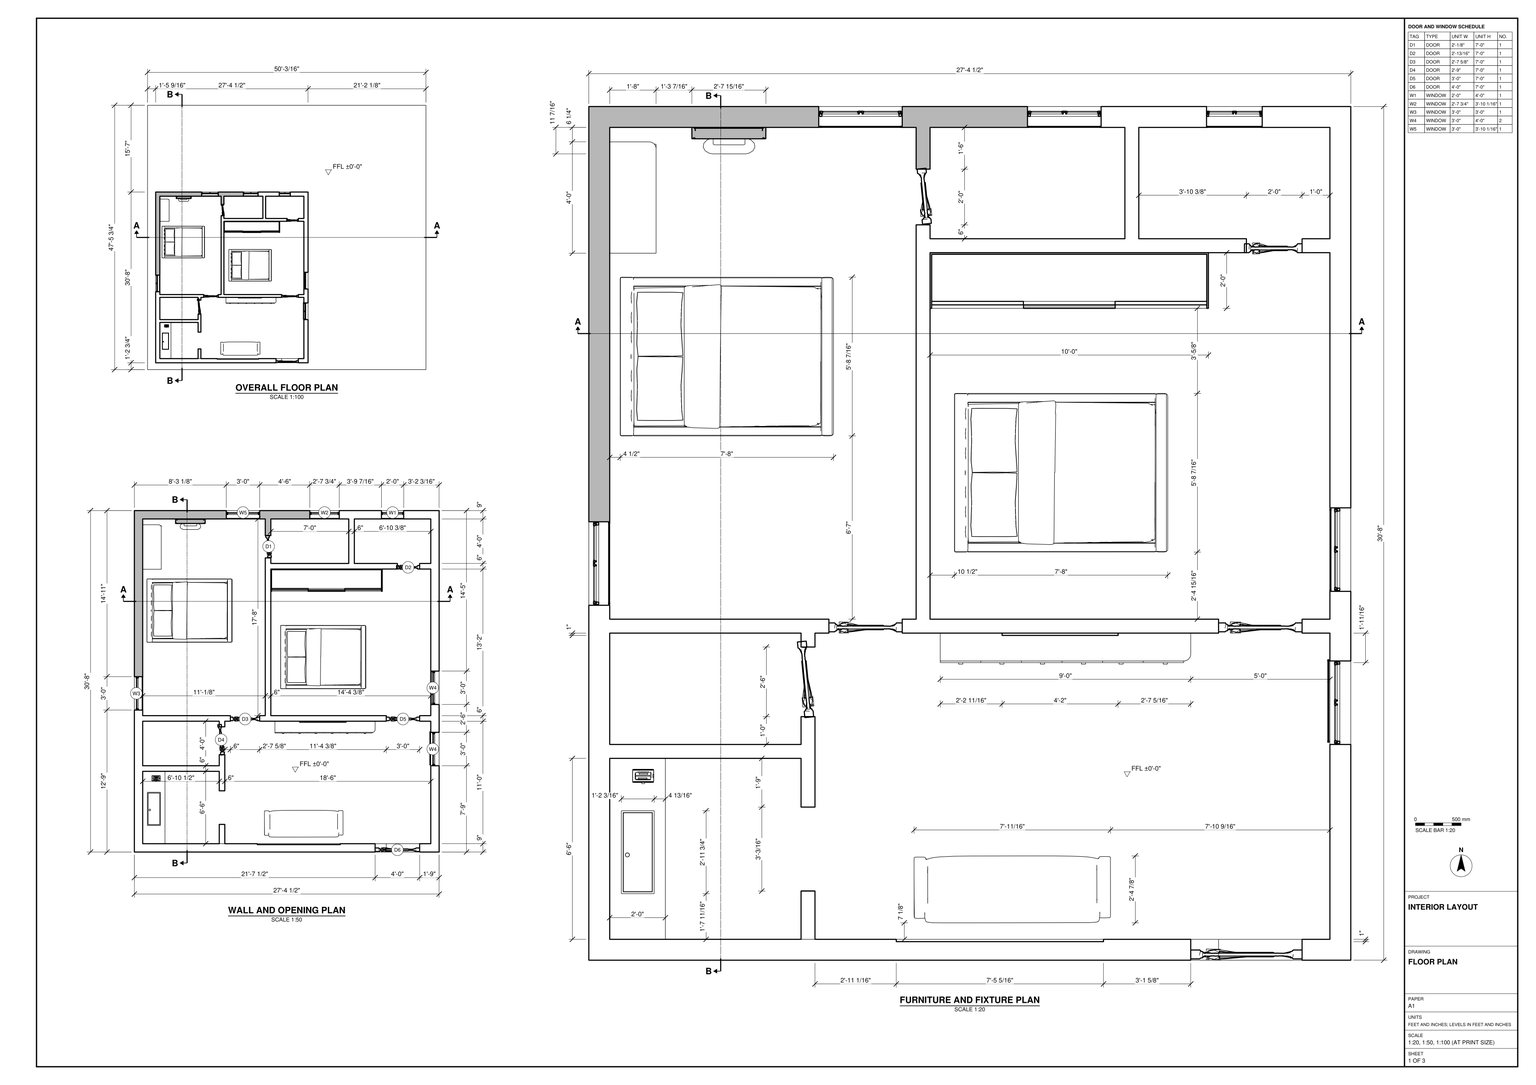
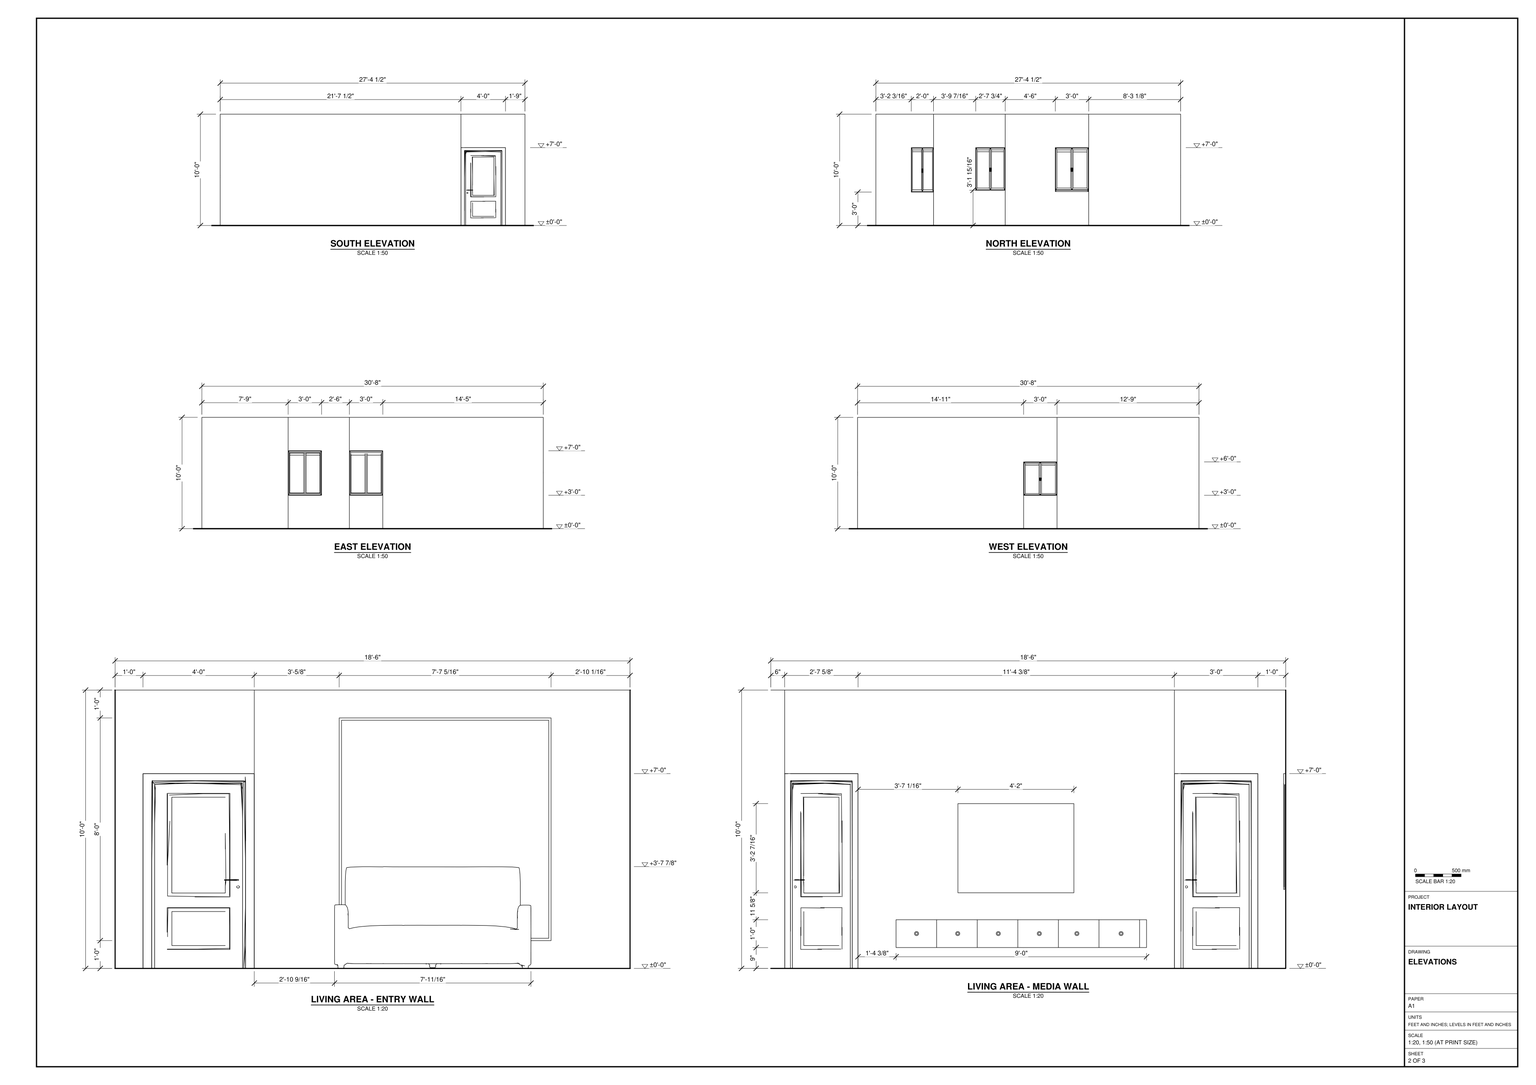
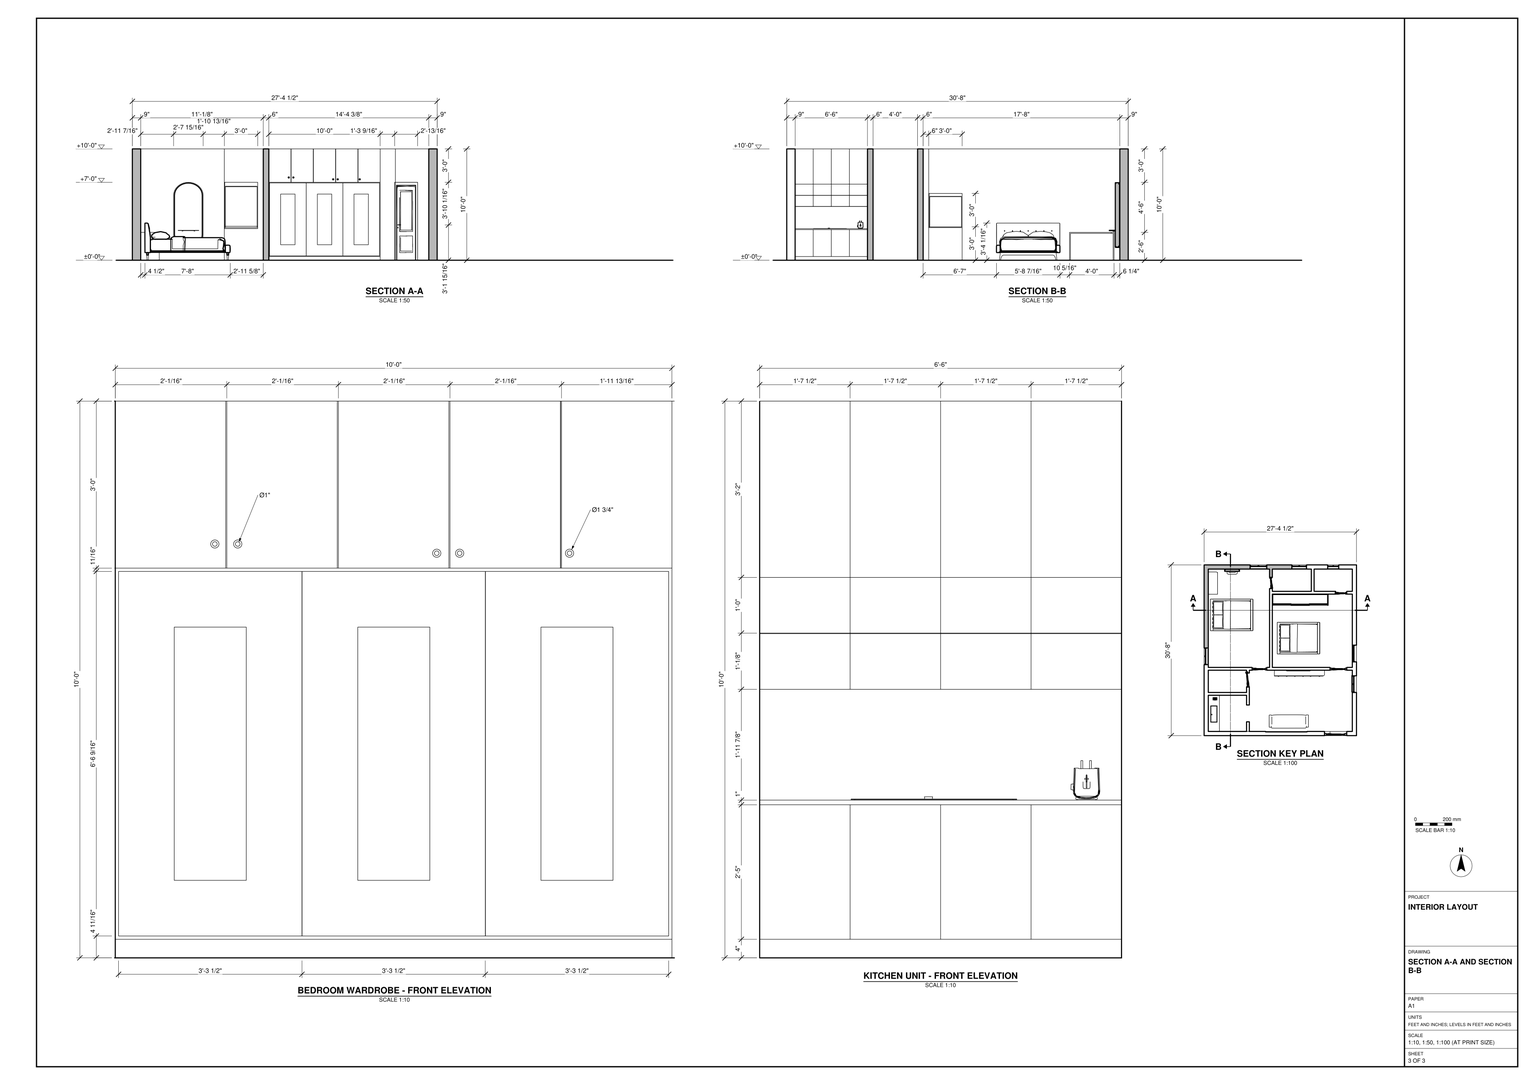
Build the interior in SketchUp from task_files/diagram_01.pdf. Work in feet and inches. The overall model measures 50'-3/16" east to west by 47'-5 3/4" north to south and is 10'-0" high. Set the finished floor at ±0'-0". Use the overall floor plan to position the 27'-4 1/2" by 30'-8" enclosure on the larger floor area; the enclosure and the floor have different footprints.

Build the 9" perimeter walls and 6" internal partitions as drawn. Lay out the two bedrooms, the small enclosed spaces and the living area with its adjoining kitchen. Use the plan and schedule for door and window sizes and positions, and the elevations for sill and head heights.

Place a platform bed in each bedroom with its head to the west. Use the joinery elevations to model the wardrobe in the east bedroom and the kitchen unit along the west wall, including cabinet divisions, the worktop and the cooktop. Place the sofa against the entry wall, with the wall panel behind it, facing the media unit between the bedroom doors. Decor and loose items, including countertop appliances, may be any suitable library components.

Keep shell elements and individual furniture and joinery pieces in separate groups or components, and use components for repeated parts. Save one SketchUp model as output_files/furnished_two_bedroom_interior_with_built_in_joinery.skp.

# SketchUp Ruby script. Lengths in inches.
U = 1.inch
M = Sketchup.active_model
def pt(a) = Geom::Point3d.new(a.map { |v| v * U })
def face(e, loops, mat)
  f = e.add_face(loops[0].map { |a| pt(a) })
  loops[1..].each { |l| e.add_face(l.map { |a| pt(a) }).erase! }
  f.material = f.back_material = mat if mat
  f
end
# faces: each face lists its corners as indices into pts; further lists are holes
def faces(e, pts, list, mat = nil) = list.each { |f| face(e, (f[0].is_a?(Array) ? f : [f]).map { |l| l.map { |i| pts[i] } }, mat) }
# xy, xz, yz: faces in a plane at the given z, y or x. An outline is a flat list of corners, or four numbers for a rectangle; further outlines are holes
def ring(l) = l.size == 4 ? [[l[0], l[1]], [l[2], l[1]], [l[2], l[3]], [l[0], l[3]]] : l.each_slice(2).to_a
def flat(e, list, mat, &to3) = list.each { |f| face(e, (f[0].is_a?(Array) ? f : [f]).map { |l| ring(l).map { |u, v| to3.(u, v) } }, mat) }
def xy(e, z, list, mat = nil) = flat(e, list, mat) { |x, y| [x, y, z] }
def xz(e, y, list, mat = nil) = flat(e, list, mat) { |x, z| [x, y, z] }
def yz(e, x, list, mat = nil) = flat(e, list, mat) { |y, z| [x, y, z] }
def lines(e, pts, list) = list.each { |a, b| e.add_line(pt(pts[a]), pt(pts[b])) }
# prism: a flat outline (further loops are holes) pulled along v
def prism(e, loops, v, mat = nil)
  f = face(e, loops, mat); d = Geom::Vector3d.new(v.map { |x| x * U })
  f.pushpull(f.normal.samedirection?(d) ? d.length : -d.length)
end
def box(e, o, s, mat = nil) = prism(e, [[o, [o[0] + s[0], o[1], o[2]], [o[0] + s[0], o[1] + s[1], o[2]], [o[0], o[1] + s[1], o[2]]]], [0, 0, s[2]], mat)
def at(x, y, z, deg = 0) = Geom::Transformation.translation(pt([x, y, z])) * Geom::Transformation.rotation(ORIGIN, Z_AXIS, deg.degrees)
def axes(o, x, y, z) = Geom::Transformation.new([*x, 0, *y, 0, *z, 0, *pt(o).to_a, 1])
def part(name) = M.definitions.add(name)
# library, detail: a bought-in or finely detailed component or shape, given as its bounding box
def library(name, o, s) = part(name).tap { |d| box(d.entities, o, s) }
def detail(e, o, s) = box(e.add_group.entities, o, s)
def put(e, d, t, mat = nil) = e.add_instance(d, t).tap { |i| i.material = mat if mat }
def group(e, t, mat = nil) = e.add_group.tap { |g| g.transformation = t; g.material = mat if mat }.entities
root = M.entities
M.materials.add("[0007_MistyRose]").color = [255, 228, 225]
M.materials.add("[Aluminum]").color = [229, 229, 229]
M.materials.add("[Color D01]").color = [255, 242, 204]
M.materials.add("[Color M00]").color = [255, 255, 255]
M.materials.add("[Color M01]").color = [226, 226, 226]
M.materials.add("[Color M02]").color = [198, 198, 198]
M.materials.add("[Color M09]").color = [0, 0, 0]
M.materials.add("[Marble Carrara Gold Floor Tile]").color = [225, 223, 217]
c1 = library("Sofa 142 022",[-42.35,-14.43,0],[84.7,28.86,43.89])
c2 = library("Katherine Ring Wall",[-15.98,-14.97,0],[31.92,14.82,81.1])
c3 = library("Door 243 074",[-20.11,-2.41,0],[40.22,4.82,86.63])
c4 = library("Window 46-10",[-43.56,-2.12,0],[87.13,4.27,82.67])
c5 = library("Tyler Platform Bed",[-34.22,-45.98,0],[68.44,91.98,40.05])
c6 = part("Shutters 01 47-19")
xy(c6.entities,0,[[-41.74,2.35,-43.47,3.54,-41.74,3.54],[-43.47,2.35,-43.47,3.54,-41.74,2.35],[-41.74,2.35,-41.74,3.54,41.72,3.54],[-41.74,2.35,41.72,3.54,41.72,2.35],[41.72,2.35,41.72,3.54,43.47,2.35],
  [43.47,2.35,41.72,3.54,43.47,3.54]])
xy(c6.entities,1.4,[[-41.74,2.35,41.72,2.35,-41.74,3.54],[41.72,2.35,41.72,3.54,-41.74,3.54],[-41.74,2.51,-41.74,3.39,41.72,3.39],[-41.74,2.51,41.72,3.39,41.72,2.51]])
xy(c6.entities,59.85,[[-43.47,-1.5625,-41.74,2.35,-41.74,-1.5625],[-43.47,-1.5625,-43.47,2.35,-41.74,2.35],[-41.74,-1.5625,-41.74,2.35,41.72,2.35],[-41.74,-1.5625,41.72,2.35,41.72,-1.5625],[41.72,-1.5625,41.72,2.35,43.47,2.35],
  [41.72,-1.5625,43.47,2.35,43.47,-1.5625],[-41.74,2.35,-41.74,3.54,41.72,3.54],[-41.74,2.35,41.72,3.54,41.72,2.35]])
xy(c6.entities,60.45,[[-41.74,2.51,41.72,2.51,41.72,3.39],[-41.74,2.51,41.72,3.39,-41.74,3.39]])
xy(c6.entities,66.14,[[-41.74,-3.54,-41.74,2.35,-43.47,2.35],[-43.47,-3.54,-41.74,-3.54,-43.47,2.35],[-41.74,-3.54,41.72,-3.54,-41.74,2.35],[41.72,-3.54,41.72,2.35,-41.74,2.35],[41.72,-3.54,43.47,-3.54,41.72,2.35],
  [43.47,-3.54,43.47,2.35,41.72,2.35],[-43.47,2.35,-41.74,2.35,-41.74,3.54],[-43.47,2.35,-41.74,3.54,-43.47,3.54],[-41.74,2.35,41.72,2.35,41.72,3.54],[-41.74,2.35,41.72,3.54,-41.74,3.54],
  [41.72,2.35,43.47,2.35,43.47,3.54],[41.72,2.35,43.47,3.54,41.72,3.54]])
xz(c6.entities,-3.54,[[-41.74,61.84,-41.74,66.14,-43.47,66.14],[-43.47,61.84,-41.74,61.84,-43.47,66.14],[-41.74,61.84,41.72,61.84,-41.74,66.14],[41.72,61.84,41.72,66.14,-41.74,66.14],[41.72,61.84,43.47,61.84,41.72,66.14],
  [43.47,61.84,43.47,66.14,41.72,66.14]])
xz(c6.entities,2.35,[[-43.47,0,-41.74,0,-41.74,1.4],[-43.47,0,-41.74,1.4,-43.47,1.4],[-41.74,0,41.72,0,-41.74,1.4],[41.72,0,41.72,1.4,-41.74,1.4],[41.72,0,43.47,0,43.47,1.4],
  [41.72,0,43.47,1.4,41.72,1.4],[-41.74,1.4,-41.74,59.85,-43.47,59.85],[-43.47,1.4,-41.74,1.4,-43.47,59.85],[41.72,1.4,43.47,1.4,41.72,59.85],[43.47,1.4,43.47,59.85,41.72,59.85]])
xz(c6.entities,2.51,[[-41.74,1.4,41.72,1.4,41.72,60.45],[-41.74,1.4,41.72,60.45,-41.74,60.45]])
xz(c6.entities,3.39,[[-41.74,1.4,-41.74,60.45,41.72,1.4],[41.72,1.4,-41.74,60.45,41.72,60.45]])
xz(c6.entities,3.54,[[-41.74,0,-43.47,1.4,-41.74,1.4],[-43.47,0,-43.47,1.4,-41.74,0],[-41.74,0,-41.74,1.4,41.72,1.4],[-41.74,0,41.72,1.4,41.72,0],[41.72,0,41.72,1.4,43.47,0],
  [43.47,0,41.72,1.4,43.47,1.4],[-43.47,1.4,-41.74,59.85,-41.74,1.4],[-43.47,1.4,-43.47,59.85,-41.74,59.85],[41.72,1.4,41.72,59.85,43.47,59.85],[41.72,1.4,43.47,59.85,43.47,1.4],
  [-43.47,59.85,-41.74,61.84,-41.74,59.85],[-43.47,59.85,-43.47,61.84,-41.74,61.84],[-41.74,59.85,-41.74,61.84,41.72,61.84],[-41.74,59.85,41.72,61.84,41.72,59.85],[41.72,59.85,41.72,61.84,43.47,61.84],
  [41.72,59.85,43.47,61.84,43.47,59.85],[-43.47,61.84,-41.74,66.14,-41.74,61.84],[-43.47,61.84,-43.47,66.14,-41.74,66.14],[-41.74,61.84,-41.74,66.14,41.72,66.14],[-41.74,61.84,41.72,66.14,41.72,61.84],
  [41.72,61.84,41.72,66.14,43.47,66.14],[41.72,61.84,43.47,66.14,43.47,61.84]])
yz(c6.entities,-43.47,[[2.35,0,2.35,1.4,3.54,0],[3.54,0,2.35,1.4,3.54,1.4],[2.35,1.4,2.35,59.85,3.54,59.85],[2.35,1.4,3.54,59.85,3.54,1.4],[-1.5625,59.85,-3.54,61.84,2.35,61.84],
  [-1.5625,59.85,2.35,61.84,2.35,59.85],[2.35,59.85,2.35,61.84,3.54,61.84],[2.35,59.85,3.54,61.84,3.54,59.85],[-3.54,61.84,-3.54,66.14,2.35,61.84],[2.35,61.84,-3.54,66.14,2.35,66.14],
  [2.35,61.84,2.35,66.14,3.54,61.84],[3.54,61.84,2.35,66.14,3.54,66.14]])
yz(c6.entities,-41.74,[[2.35,1.4,3.54,1.4,2.35,59.85],[3.54,1.4,3.54,59.85,2.35,59.85],[2.51,1.4,2.51,60.45,3.39,1.4],[3.39,1.4,2.51,60.45,3.39,60.45]])
yz(c6.entities,41.72,[[2.35,1.4,2.35,59.85,3.54,59.85],[2.35,1.4,3.54,59.85,3.54,1.4],[2.51,1.4,3.39,1.4,3.39,60.45],[2.51,1.4,3.39,60.45,2.51,60.45]])
yz(c6.entities,43.47,[[2.35,0,3.54,0,3.54,1.4],[2.35,0,3.54,1.4,2.35,1.4],[2.35,1.4,3.54,1.4,2.35,59.85],[3.54,1.4,3.54,59.85,2.35,59.85],[-1.5625,59.85,2.35,61.84,-3.54,61.84],
  [-1.5625,59.85,2.35,59.85,2.35,61.84],[2.35,59.85,3.54,59.85,2.35,61.84],[3.54,59.85,3.54,61.84,2.35,61.84],[-3.54,61.84,2.35,61.84,-3.54,66.14],[2.35,61.84,2.35,66.14,-3.54,66.14],
  [2.35,61.84,3.54,61.84,3.54,66.14],[2.35,61.84,3.54,66.14,2.35,66.14]])
p = [[-43.47,-3.54,61.84],[-43.47,-1.5625,59.85],[-41.74,-1.5625,59.85],[-41.74,-3.54,61.84],[41.72,-1.5625,59.85],[41.72,-3.54,61.84],
  [43.47,-1.5625,59.85],[43.47,-3.54,61.84]]
faces(c6.entities,p,[[0,1,2],[2,3,0],[4,5,3],[3,2,4],[6,7,5],[5,4,6]])
c7 = library("Toaster 145 006",[-4.61,-3.12,0],[9.22,6.24,8.52])
c8 = library("Induction Hob 33-08",[-17.875,-7.09,0.04],[35.75,14.18,0.72])
c9 = part("Group\#11")
box(c9.entities,[0.2,0,0],[23.8,0.71,36])
c10 = part("Group\#14")
box(c10.entities,[0,0,0],[17.5,0.71,12])
c11 = part("Group\#19")
xy(c11.entities,0,[[3.125,0,2.32,0.11,1.5625,0.42,0.92,0.92,0.42,1.5625,0.11,2.32,0,3.125,0.11,3.93,0.42,4.6875,0.92,5.33,1.5625,5.83,2.32,6.14,3.125,6.25,3.93,6.14,4.6875,5.83,5.33,5.33,5.83,4.6875,6.14,3.93,6.25,3.125,6.14,2.32,5.83,1.5625,5.33,0.92,4.6875,0.42,3.93,0.11]],"[Color M09]")
xy(c11.entities,0.375,[[3.125,1.37,3.58,1.43,4,1.61,4.36,1.89,4.64,2.25,4.82,2.67,4.88,3.125,4.82,3.58,4.64,4,4.36,4.36,4,4.64,3.58,4.82,3.125,4.88,2.67,4.82,2.25,4.64,1.89,4.36,1.61,4,1.43,3.58,1.37,3.125,1.43,2.67,1.61,2.25,1.89,1.89,2.25,1.61,2.67,1.43]],"[Color M09]")
xy(c11.entities,1,[[[3.125,0,3.93,0.11,4.6875,0.42,5.33,0.92,5.83,1.5625,6.14,2.32,6.25,3.125,6.14,3.93,5.83,4.6875,5.33,5.33,4.6875,5.83,3.93,6.14,3.125,6.25,2.32,6.14,1.5625,5.83,0.92,5.33,0.42,4.6875,0.11,3.93,0,3.125,0.11,2.32,0.42,1.5625,0.92,0.92,1.5625,0.42,2.32,0.11],[3.125,1.37,2.67,1.43,2.25,1.61,1.89,1.89,1.61,2.25,1.43,2.67,1.37,3.125,1.43,3.58,1.61,4,1.89,4.36,2.25,4.64,2.67,4.82,3.125,4.88,3.58,4.82,4,4.64,4.36,4.36,4.64,4,4.82,3.58,4.88,3.125,4.82,2.67,4.64,2.25,4.36,1.89,4,1.61,3.58,1.43]]],"[Color M09]")
p = [[2.32,0.11,0],[3.125,0,0],[3.125,0,1],[2.32,0.11,1],[3.93,0.11,0],[3.93,0.11,1],
  [1.5625,0.42,0],[1.5625,0.42,1],[4.6875,0.42,0],[4.6875,0.42,1],[0.92,0.92,0],[0.92,0.92,1],
  [5.33,0.92,0],[5.33,0.92,1],[0.42,1.5625,0],[0.42,1.5625,1],[5.83,1.5625,0],[5.83,1.5625,1],
  [0.11,2.32,0],[0.11,2.32,1],[6.14,2.32,0],[6.14,2.32,1],[0,3.125,0],[0,3.125,1],
  [6.25,3.125,0],[6.25,3.125,1],[0.11,3.93,0],[0.11,3.93,1],[6.14,3.93,0],[6.14,3.93,1],
  [0.42,4.6875,0],[0.42,4.6875,1],[5.83,4.6875,0],[5.83,4.6875,1],[0.92,5.33,0],[0.92,5.33,1],
  [5.33,5.33,0],[5.33,5.33,1],[1.5625,5.83,0],[1.5625,5.83,1],[4.6875,5.83,0],[4.6875,5.83,1],
  [2.32,6.14,0],[2.32,6.14,1],[3.93,6.14,0],[3.93,6.14,1],[3.125,6.25,0],[3.125,6.25,1],
  [2.25,1.61,1],[2.67,1.43,1],[2.67,1.43,0.375],[2.25,1.61,0.375],[3.125,1.37,1],[3.125,1.37,0.375],
  [3.58,1.43,1],[3.58,1.43,0.375],[4,1.61,1],[4,1.61,0.375],[1.89,1.89,1],[1.89,1.89,0.375],
  [4.36,1.89,1],[4.36,1.89,0.375],[1.61,2.25,1],[1.61,2.25,0.375],[4.64,2.25,1],[4.64,2.25,0.375],
  [1.43,2.67,1],[1.43,2.67,0.375],[4.82,2.67,1],[4.82,2.67,0.375],[1.37,3.125,1],[1.37,3.125,0.375],
  [4.88,3.125,1],[4.88,3.125,0.375],[1.43,3.58,1],[1.43,3.58,0.375],[4.82,3.58,1],[4.82,3.58,0.375],
  [1.61,4,1],[1.61,4,0.375],[4.64,4,1],[4.64,4,0.375],[1.89,4.36,1],[1.89,4.36,0.375],
  [4.36,4.36,1],[4.36,4.36,0.375],[2.25,4.64,1],[2.25,4.64,0.375],[4,4.64,1],[4,4.64,0.375],
  [2.67,4.82,1],[2.67,4.82,0.375],[3.58,4.82,1],[3.58,4.82,0.375],[3.125,4.88,1],[3.125,4.88,0.375]]
faces(c11.entities,p,[[0,1,2,3],[1,4,5,2],[6,0,3,7],[4,8,9,5],[10,6,7,11],[8,12,13,9],[14,10,11,15],[12,16,17,13],
  [18,14,15,19],[16,20,21,17],[22,18,19,23],[20,24,25,21],[26,22,23,27],[24,28,29,25],[30,26,27,31],[28,32,33,29],
  [34,30,31,35],[32,36,37,33],[38,34,35,39],[36,40,41,37],[42,38,39,43],[40,44,45,41],[46,42,43,47],[44,46,47,45],
  [48,49,50,51],[49,52,53,50],[52,54,55,53],[54,56,57,55],[58,48,51,59],[56,60,61,57],[62,58,59,63],[60,64,65,61],
  [66,62,63,67],[64,68,69,65],[70,66,67,71],[68,72,73,69],[74,70,71,75],[72,76,77,73],[78,74,75,79],[76,80,81,77],
  [82,78,79,83],[80,84,85,81],[86,82,83,87],[84,88,89,85],[90,86,87,91],[88,92,93,89],[94,90,91,95],[92,94,95,93]],"[Color M09]")
c12 = part("Group\#20")
box(c12.entities,[0,0,0],[0.71,19.5,12])
c13 = part("Group\#18")
box(c13.entities,[0,0,0],[0.71,19.5,38])
xy(root,0,[[17.5625,14.75,277.0625,14.75,277.0625,23.75,26.5625,23.75,26.5625,101.75,109.0625,101.75,109.0625,80.75,115.0625,80.75,115.0625,119.75,109.0625,119.75,109.0625,107.75,26.5625,107.75,26.5625,155.75,109.0625,155.75,109.0625,149.75,115.0625,149.75,115.0625,155.75,121.0625,155.75,121.0625,161.75,26.5625,161.75,26.5625,167.75,17.5625,167.75],[277.0625,14.75,289.0625,23.75],[289.0625,14.75,325.0625,23.75],[325.0625,14.75,346.0625,14.75,346.0625,107.75,337.0625,107.75,337.0625,23.75,325.0625,23.75],[109.0625,23.75,115.0625,44.75],
  [337.0625,143.75,346.0625,143.75,346.0625,173.75,337.0625,173.75,337.0625,161.75,325.0625,161.75,325.0625,155.75,337.0625,155.75],[152.67,155.75,289.0625,155.75,289.0625,161.75,164.67,161.75,164.67,319.75,301.0625,319.75,301.0625,325.75,254.67,325.75,254.67,373.75,283.87,373.75,283.87,382.75,238.42,382.75,238.42,373.75,248.67,373.75,248.67,325.75,164.67,325.75,164.67,331.75,158.67,331.75,158.67,161.75,152.67,161.75],[17.5625,167.75,26.5625,203.75],[337.0625,173.75,346.0625,209.75],[17.5625,203.75,26.5625,203.75,26.5625,373.75,116.67,373.75,116.67,382.75,17.5625,382.75],
  [337.0625,209.75,346.0625,209.75,346.0625,382.75,307.87,382.75,307.87,373.75,337.0625,373.75,337.0625,325.75,325.0625,325.75,325.0625,319.75,337.0625,319.75],[164.67,295.75,284.67,319.75],[158.67,355.75,164.67,355.75,164.67,373.75,206.67,373.75,206.67,382.75,152.67,382.75,152.67,373.75,158.67,373.75],[116.67,373.75,152.67,382.75],[206.67,373.75,238.42,382.75],
  [283.87,373.75,307.87,382.75]])
xy(root,0,[[[0,0,600.19,569.75],[17.5625,14.75,346.0625,382.75]]],"[Color M00]")
xy(root,0,[[26.5625,23.75,109.0625,23.75,109.0625,44.75,115.0625,44.75,115.0625,23.75,337.0625,23.75,337.0625,107.75,346.0625,107.75,346.0625,143.75,337.0625,143.75,337.0625,155.75,325.0625,155.75,325.0625,161.75,337.0625,161.75,337.0625,319.75,325.0625,319.75,325.0625,325.75,337.0625,325.75,337.0625,373.75,254.67,373.75,254.67,325.75,301.0625,325.75,301.0625,319.75,284.67,319.75,284.67,295.75,164.67,295.75,164.67,161.75,289.0625,161.75,289.0625,155.75,152.67,155.75,152.67,161.75,158.67,161.75,158.67,331.75,164.67,331.75,164.67,325.75,248.67,325.75,248.67,373.75,164.67,373.75,164.67,355.75,158.67,355.75,158.67,373.75,26.5625,373.75,26.5625,161.75,121.0625,161.75,121.0625,155.75,115.0625,155.75,115.0625,149.75,109.0625,149.75,109.0625,155.75,26.5625,155.75,26.5625,107.75,109.0625,107.75,109.0625,119.75,115.0625,119.75,115.0625,80.75,109.0625,80.75,109.0625,101.75,26.5625,101.75]],"[Marble Carrara Gold Floor Tile]")
xy(root,36,[[17.5625,167.75,26.5625,203.75],[337.0625,173.75,346.0625,209.75]])
xy(root,84,[[277.0625,14.75,325.0625,23.75]])
xy(root,120,[[277.0625,14.75,346.0625,14.75,346.0625,107.75,337.0625,107.75,337.0625,23.75,277.0625,23.75]])
xz(root,14.75,[[325.0625,0,346.0625,0,346.0625,120,277.0625,120,277.0625,84,325.0625,84]])
xz(root,23.75,[[325.0625,0,325.0625,84,277.0625,84,277.0625,120,337.0625,120,337.0625,0]])
xz(root,107.75,[[337.0625,0,346.0625,120]])
xz(root,167.75,[[17.5625,0,26.5625,36]])
xz(root,173.75,[[337.0625,0,346.0625,36]])
xz(root,203.75,[[17.5625,0,26.5625,36]])
xz(root,209.75,[[337.0625,0,346.0625,36]])
yz(root,17.5625,[[167.75,0,203.75,36]])
yz(root,26.5625,[[167.75,0,203.75,36]])
yz(root,277.0625,[[14.75,84,23.75,120]])
yz(root,325.0625,[[14.75,0,23.75,84]])
yz(root,337.0625,[[23.75,0,107.75,120],[173.75,0,209.75,36]])
yz(root,346.0625,[[14.75,0,107.75,120],[173.75,0,209.75,36]])
p = [[169.0625,155.75,0],[169.0625,143.75,0],[600.19,0,0],[915.125,0,0]]
lines(root,p,[[0,1],[2,3]])
put(root,c1,at(200.125,45.28,0,-180))
put(root,c2,axes([77.95,373.86,13.44],[1,0,0],[0,0.77,0],[0,0,0.87]))
put(root,c3,axes([307.0625,158.16,0],[0.8949,0,0],[0,1,0],[0,0,0.9696]))
put(root,c3,axes([312.64,321.59,0],[0.61748,0,0],[0,1,0],[0,0,0.9696]))
put(root,c3,axes([111.07,135.82,0],[-0.07948,0.81062,0],[-0.99523,-0.09758,0],[0,0,0.9696]))
put(root,c3,axes([162.24,344.1,0],[-0.05794,0.59092,0],[-0.99523,-0.09758,0],[0,0,0.9696]))
put(root,c3,axes([301.0625,17.16,0],[1.1932,0,0],[0,1,0],[0,0,0.9696]))
put(root,c4,axes([19.68,185.75,36],[0,-0.41317,0],[1,0,0],[0,0,0.43546]))
put(root,c4,axes([339.18,125.75,36],[0,-0.41317,0],[1,0,0],[0,0,0.58062]))
put(root,c4,axes([339.18,191.75,36],[0,-0.41317,0],[1,0,0],[0,0,0.58062]))
put(root,c4,axes([222.55,380.63,37.95],[-0.3644,0,0],[0,-1,0],[0,0,0.55697]))
put(root,c4,axes([295.87,380.63,36],[-0.27545,0,0],[0,-1,0],[0,0,0.58062]))
put(root,c4,axes([134.67,380.63,37.95],[-0.41317,0,0],[0,-1,0],[0,0,0.55697]))
put(root,c5,at(221.17,224.89,0,90))
put(root,c5,at(77.07,274.96,0,90))
put(root,c3,axes([136.87,158.16,0],[0.78577,0,0],[0,1,0],[0,0,0.9696]))
put(root,c6,axes([337.58,126.49,34.06],[0,0.40872,0],[-0.4,0,0],[0,0,0.75509]))
put(root,c6,axes([338.48,191.52,34.06],[0,0.40872,0],[-0.4,0,0],[0,0,0.75509]))
put(root,c6,axes([134.91,375.17,34.06],[-0.40872,0,0],[0,-0.4,0],[0,0,0.75509]))
put(root,c6,axes([222.55,375.17,37.3],[-0.36523,0,0],[0,-0.4,0],[0,0,0.70599]))
put(root,c6,axes([295.87,375.17,37.3],[-0.27608,0,0],[0,-0.4,0],[0,0,0.70599]))
put(root,c6,axes([25.15,185.98,35.15],[0,-0.40872,0],[0.4,0,0],[0,0,0.55719]))
put(root,c7,at(41,93.97,34))
put(root,c8,at(38.66,61.31,33.96,-90))
g1 = group(root,at(17.5625,203.75,0))
xy(g1,0,[[0,0,0,179,99.11,179,99.11,170,9,170,9,0]])
xy(g1,72,[[0,-36,9,0]])
xy(g1,120,[[0,-36,9,-36,9,170,99.11,170,99.11,179,0,179]])
xz(g1,-36,[[0,72,9,120]])
xz(g1,0,[[0,0,9,72]])
xz(g1,170,[[9,0,99.11,120]])
xz(g1,179,[[0,0,99.11,120]])
yz(g1,0,[[0,0,0,72,-36,72,-36,120,179,120,179,0]])
yz(g1,9,[[0,0,170,0,170,120,-36,120,-36,72,0,72]])
yz(g1,99.11,[[170,0,179,120]])
g2 = group(root,at(152.67,355.75,0))
xy(g2,0,[[6,0,6,18,-36,18,-36,27,54,27,54,18,12,18,12,0]])
xy(g2,36.59,[[-36,18,0,27]])
xy(g2,84,[[6,-24,12,0],[-36,18,0,27]])
xy(g2,120,[[6,-24,12,-24,12,18,54,18,54,27,-36,27,-36,18,6,18]])
xz(g2,-24,[[6,84,12,120]])
xz(g2,0,[[6,0,12,84]])
xz(g2,18,[[-36,0,6,0,6,120,-36,120,-36,84,0,84,0,36.59,-36,36.59],[12,0,54,120]])
xz(g2,27,[[-36,0,-36,36.59,0,36.59,0,84,-36,84,-36,120,54,120,54,0]])
yz(g2,-36,[[18,0,27,36.59],[18,84,27,120]])
yz(g2,0,[[18,36.59,27,84]])
yz(g2,6,[[0,0,0,84,-24,84,-24,120,18,120,18,0]])
yz(g2,12,[[0,0,18,0,18,120,-24,120,-24,84,0,84]])
yz(g2,54,[[18,0,27,120]])
g3 = group(root,at(307.87,209.75,0))
xy(g3,0,[[29.19,0,29.19,110,17.19,110,17.19,116,29.19,116,29.19,164,-24,164,-24,173,38.19,173,38.19,0]])
xy(g3,36,[[-24,164,0,173]])
xy(g3,84,[[29.19,-36,38.19,0],[-6.81,110,17.19,116],[-24,164,0,173]])
xy(g3,120,[[29.19,-36,38.19,-36,38.19,173,-24,173,-24,164,29.19,164,29.19,116,-6.81,116,-6.81,110,29.19,110]])
xz(g3,-36,[[29.19,84,38.19,120]])
xz(g3,0,[[29.19,0,38.19,84]])
xz(g3,110,[[17.19,0,29.19,0,29.19,120,-6.81,120,-6.81,84,17.19,84]])
xz(g3,116,[[17.19,0,17.19,84,-6.81,84,-6.81,120,29.19,120,29.19,0]])
xz(g3,164,[[-24,0,29.19,0,29.19,120,-24,120,-24,84,0,84,0,36,-24,36]])
xz(g3,173,[[-24,0,-24,36,0,36,0,84,-24,84,-24,120,38.19,120,38.19,0]])
yz(g3,-24,[[164,0,173,36],[164,84,173,120]])
yz(g3,-6.81,[[110,84,116,120]])
yz(g3,0,[[164,36,173,84]])
yz(g3,17.19,[[110,0,116,84]])
yz(g3,29.19,[[0,0,0,84,-36,84,-36,120,110,120,110,0],[116,0,164,120]])
yz(g3,38.19,[[0,0,173,0,173,120,-36,120,-36,84,0,84]])
g4 = group(root,at(152.67,155.75,0))
xy(g4,0,[[0,0,0,6,6,6,6,176,12,176,12,170,96,170,96,218,54,218,54,227,131.2,227,131.2,218,102,218,102,170,148.39,170,148.39,164,12,164,12,6,136.39,6,136.39,0]])
xy(g4,37.95,[[54,218,85.75,227]])
xy(g4,84,[[-31.61,0,0,6],[54,218,85.75,227]])
xy(g4,120,[[-31.61,0,136.39,0,136.39,6,12,6,12,164,148.39,164,148.39,170,102,170,102,218,131.2,218,131.2,227,54,227,54,218,96,218,96,170,12,170,12,176,6,176,6,6,-31.61,6]])
xz(g4,0,[[[0,0,136.39,0,136.39,120,-31.61,120,-31.61,84,0,84],[43.07,32.61,93.07,71.05]],[43.07,32.61,93.07,71.05]])
xz(g4,6,[[0,0,0,84,-31.61,84,-31.61,120,6,120,6,0],[12,0,136.39,120]])
xz(g4,164,[[12,0,148.39,120]])
xz(g4,170,[[12,0,96,120],[102,0,148.39,120]])
xz(g4,176,[[6,0,12,120]])
xz(g4,218,[[54,0,96,0,96,120,54,120,54,84,85.75,84,85.75,37.95,54,37.95],[102,0,131.2,120]])
xz(g4,227,[[54,0,54,37.95,85.75,37.95,85.75,84,54,84,54,120,131.2,120,131.2,0]])
yz(g4,-31.61,[[0,84,6,120]])
yz(g4,0,[[0,0,6,84]])
yz(g4,6,[[6,0,176,120]])
yz(g4,12,[[6,0,164,120],[170,0,176,120]])
yz(g4,54,[[218,0,227,37.95],[218,84,227,120]])
yz(g4,85.75,[[218,37.95,227,84]])
yz(g4,96,[[170,0,218,120]])
yz(g4,102,[[170,0,218,120]])
yz(g4,131.2,[[218,0,227,120]])
yz(g4,136.39,[[0,0,6,120]])
yz(g4,148.39,[[164,0,170,120]])
g5 = group(g4,at(43.07,-1,32.61),"[Color M09]")
box(g5,[0,0,0],[50,1,38.4375])
g6 = group(root,at(325.0625,143.75,0))
xy(g6,0,[[12,-36,12,12,0,12,0,18,12,18,12,30,21,30,21,-36]])
xy(g6,36,[[12,-36,21,0]])
xy(g6,84,[[12,-36,21,0],[-36,12,0,18]])
xy(g6,120,[[12,-36,21,-36,21,30,12,30,12,18,-36,18,-36,12,12,12]])
xz(g6,-36,[[12,0,21,36],[12,84,21,120]])
xz(g6,0,[[12,36,21,84]])
xz(g6,12,[[0,0,12,0,12,120,-36,120,-36,84,0,84]])
xz(g6,18,[[0,0,0,84,-36,84,-36,120,12,120,12,0]])
xz(g6,30,[[12,0,21,120]])
yz(g6,-36,[[12,84,18,120]])
yz(g6,0,[[12,0,18,84]])
yz(g6,12,[[-36,0,-36,36,0,36,0,84,-36,84,-36,120,12,120,12,0],[18,0,30,120]])
yz(g6,21,[[-36,0,30,0,30,120,-36,120,-36,84,0,84,0,36,-36,36]])
g7 = group(root,at(164.67,295.75,0),"[0007_MistyRose]")
xy(g7,0,[[0,0,120,24]])
xy(g7,4.71,[[0.71,0,119.29,1.5],[0.71,1.5,40.24,3],[40.24,1.5,79.76,3],[79.76,1.5,119.29,3],[0.71,3,119.29,23.29]])
xy(g7,83.29,[[0.71,0,119.29,23.29]])
xy(g7,84,[[0,0,120,24]])
xz(g7,0,[[0,0,120,4],[[0,4,120,84],[0.71,4.71,119.29,83.29]]])
xz(g7,23.29,[[0.71,4.71,119.29,83.29]])
xz(g7,24,[[0,0,120,84]])
yz(g7,0,[[0,0,24,84]])
yz(g7,0.71,[[0,4.71,23.29,83.29]])
yz(g7,119.29,[[0,4.71,23.29,83.29]])
yz(g7,120,[[0,0,24,84]])
g8 = group(g7,at(79.76,1.5,4.71))
xy(g8,0,[[0,0,39.53,1.5]])
xy(g8,78.58,[[0,0,39.53,1.5]])
xz(g8,0,[[[0,0,39.53,78.58],[12,12,27.53,66.58]]])
xz(g8,0,[[12,12,27.53,66.58]],"[Color D01]")
xz(g8,1.5,[[0,0,39.53,78.58]])
yz(g8,0,[[0,0,1.5,78.58]])
yz(g8,39.53,[[0,0,1.5,78.58]])
g9 = group(g7,at(40.28,0,4.71))
xy(g9,0,[[0,0,39.53,1.5]])
xy(g9,78.58,[[0,0,39.53,1.5]])
xz(g9,0,[[[0,0,39.53,78.58],[12,12,27.53,66.58]]])
xz(g9,0,[[12,12,27.53,66.58]],"[Color D01]")
xz(g9,1.5,[[0,0,39.53,78.58]])
yz(g9,0,[[0,0,1.5,78.58]])
yz(g9,39.53,[[0,0,1.5,78.58]])
g10 = group(g7,at(0.71,1.5,4.71))
xy(g10,0,[[0,0,39.53,1.5]])
xy(g10,78.58,[[0,0,39.53,1.5]])
xz(g10,0,[[[0,0,39.53,78.58],[12,12,27.53,66.58]]])
xz(g10,0,[[12,12,27.53,66.58]],"[Color D01]")
xz(g10,1.5,[[0,0,39.53,78.58]])
yz(g10,0,[[0,0,1.5,78.58]])
yz(g10,39.53,[[0,0,1.5,78.58]])
g11 = group(root,at(164.67,295.75,84),"[0007_MistyRose]")
xy(g11,0,[[0,0.71,120,24]])
xy(g11,36,[[0,0.71,120,24]])
xz(g11,0.71,[[0,0,96,36],[96,0,120,36]])
xz(g11,24,[[0,0,120,36]])
yz(g11,0,[[0.71,0,24,36]])
yz(g11,120,[[0.71,0,24,36]])
put(g11,c9,at(-0.2,0,0))
put(g11,c9,at(47.9,0,0))
put(g11,c9,at(71.95,0,0))
put(g11,c9,at(23.85,0,0))
put(g11,c9,at(96,0,0))
g12 = group(root,at(169.0625,143.75,9),"[Color M02]")
xy(g12,0,[[0,0,0,12,108,12,108,3,107.97,2.61,107.9,2.22,107.77,1.85,107.6,1.5,107.38,1.17,107.12,0.88,106.83,0.62,106.5,0.4,106.15,0.23,105.78,0.1,105.39,0.03,105,0]])
xy(g12,0.71,[[0.71,0,104.29,11.29]])
xy(g12,11.29,[[0.71,0,104.29,11.29]])
xy(g12,12,[[0,0,105,0,105.39,0.03,105.78,0.1,106.15,0.23,106.5,0.4,106.83,0.62,107.12,0.88,107.38,1.17,107.6,1.5,107.77,1.85,107.9,2.22,107.97,2.61,108,3,108,12,0,12]])
xz(g12,0,[[[0,0,105,12],[0.71,0.71,104.29,11.29]]])
xz(g12,11.29,[[0.71,0.71,104.29,11.29]])
xz(g12,12,[[0,0,108,12]])
yz(g12,0,[[0,0,12,12]])
yz(g12,0.71,[[0,0.71,11.29,11.29]])
yz(g12,104.29,[[0,0.71,11.29,11.29]])
yz(g12,108,[[3,0,12,12]])
p = [[105.39,0.03,12],[105,0,12],[105,0,0],[105.39,0.03,0],[105.78,0.1,12],[105.78,0.1,0],
  [106.15,0.23,12],[106.15,0.23,0],[106.5,0.4,12],[106.5,0.4,0],[106.83,0.62,12],[106.83,0.62,0],
  [107.12,0.88,12],[107.12,0.88,0],[107.38,1.17,12],[107.38,1.17,0],[107.6,1.5,12],[107.6,1.5,0],
  [107.77,1.85,12],[107.77,1.85,0],[107.9,2.22,12],[107.9,2.22,0],[107.97,2.61,12],[107.97,2.61,0],
  [108,3,12],[108,3,0]]
faces(g12,p,[[0,1,2,3],[4,0,3,5],[6,4,5,7],[8,6,7,9],[10,8,9,11],[12,10,11,13],[14,12,13,15],[16,14,15,17],
  [18,16,17,19],[20,18,19,21],[22,20,21,23],[24,22,23,25]])
put(g12,c10,at(0,-0.71,0))
put(g12,c10,at(17.5,-0.71,0))
put(g12,c10,at(35,-0.71,0))
put(g12,c10,at(52.5,-0.71,0))
put(g12,c10,at(70,-0.71,0))
put(g12,c10,at(87.5,-0.71,0))
g13 = group(root,at(50.5625,101.75,0,180),"[Color M01]")
xy(g13,0,[[3.59,0,24,78]],"[Color M02]")
xy(g13,4,[[0,0,3.59,78]],"[Color M02]")
xy(g13,33,[[0,0,24,78]],"[Color M02]")
xz(g13,0,[[3.59,0,24,0,24,33,0,33,0,4,3.59,4]],"[Color M02]")
xz(g13,78,[[3.59,0,3.59,4,0,4,0,33,24,33,24,0]],"[Color M02]")
yz(g13,0,[[0,4,19.5,33],[19.5,4,39,33],[39,4,58.5,33],[58.5,4,78,33]],"[Color M02]")
yz(g13,3.59,[[0,0,78,4]],"[Color M02]")
yz(g13,24,[[0,0,78,33]],"[Color M02]")
g14 = group(g13,at(0,0,33),"[Marble Carrara Gold Floor Tile]")
box(g14,[0,0,0],[24,78,1],"[Marble Carrara Gold Floor Tile]")
put(root,c11,axes([177,143.04,14.15],[0.28649,0,0],[0,0,0.28182],[0,-0.66,0]))
put(root,c11,axes([194.75,143.04,14.15],[0.28649,0,0],[0,0,0.28182],[0,-0.66,0]))
put(root,c11,axes([212.25,143.04,14.15],[0.28649,0,0],[0,0,0.28182],[0,-0.66,0]))
put(root,c11,axes([229.9375,143.04,14.15],[0.28649,0,0],[0,0,0.28182],[0,-0.66,0]))
put(root,c11,axes([246.125,143.04,14.15],[0.28649,0,0],[0,0,0.28182],[0,-0.66,0]))
put(root,c11,axes([265.1875,143.04,14.15],[0.28649,0,0],[0,0,0.28182],[0,-0.66,0]))
put(root,c11,axes([185.24,295.75,88.32],[0.28649,0,0],[0,0,0.28182],[0,-0.66,0]))
put(root,c11,axes([190.18,295.75,88.32],[0.28649,0,0],[0,0,0.28182],[0,-0.66,0]))
put(root,c11,axes([233.07,295.75,86.34],[0.28649,0,0],[0,0,0.28182],[0,-0.66,0]))
put(root,c11,axes([238.01,295.75,86.34],[0.28649,0,0],[0,0,0.28182],[0,-0.66,0]))
put(root,c11,axes([261.7,295.75,86.34],[0.28649,0,0],[0,0,0.28182],[0,-0.66,0]))
g15 = group(root,at(17.5625,14.75,0))
xy(g15,0,[[0,0,0,153,9,153,9,147,103.5,147,103.5,141,97.5,141,97.5,135,91.5,135,91.5,141,9,141,9,93,91.5,93,91.5,105,97.5,105,97.5,66,91.5,66,91.5,87,9,87,9,9,91.5,9,91.5,29.8125,97.5,29.8125,97.5,9,259.5,9,259.5,0]])
xy(g15,13,[[132.55,8,221.89,9]])
xy(g15,58,[[9,9,21,28.5],[9,28.5,21,48],[9,48,21,67.5],[9,67.5,21,87]])
xy(g15,82,[[9,9,21,28.5],[21,9,33,28.5],[9,28.5,21,48],[21,28.5,33,48],[9,48,21,67.5],
  [21,48,33,67.5],[9,67.5,21,87],[21,67.5,33,87]])
xy(g15,84,[[91.5,29.8125,97.5,66],[91.5,105,97.5,135]])
xy(g15,107,[[132.55,8,221.89,9]])
xy(g15,120,[[[0,0,259.5,0,259.5,9,97.5,9,97.5,141,103.5,141,103.5,147,9,147,9,153,0,153],[9,9,91.5,87],[9,93,91.5,141]],[9,9,33,28.5],[9,28.5,33,48],[9,48,33,67.5],[9,67.5,33,87]])
xz(g15,0,[[0,0,259.5,120]])
xz(g15,8,[[132.55,13,221.89,107]],"[Aluminum]")
xz(g15,9,[[9,0,9,58,21,58,21,82,33,82,33,120,91.5,120,91.5,0],[[97.5,0,259.5,120],[131.55,12,222.89,108]],[[131.55,12,222.89,108],[132.55,13,221.89,107]],[9,82,33,120]])
xz(g15,28.5,[[9,82,33,120]])
xz(g15,29.8125,[[91.5,0,97.5,84]])
xz(g15,48,[[9,82,33,120]])
xz(g15,66,[[91.5,0,97.5,84]])
xz(g15,67.5,[[9,82,33,120]])
xz(g15,87,[[9,0,91.5,0,91.5,120,33,120,33,82,21,82,21,58,9,58],[9,82,33,120]])
xz(g15,93,[[9,0,91.5,120]])
xz(g15,105,[[91.5,0,97.5,84]])
xz(g15,135,[[91.5,0,97.5,84]])
xz(g15,141,[[9,0,91.5,120],[97.5,0,103.5,120]])
xz(g15,147,[[9,0,103.5,120]])
xz(g15,153,[[0,0,9,120]])
yz(g15,0,[[0,0,153,120]])
yz(g15,9,[[9,0,87,58],[93,0,141,120],[147,0,153,120],[9,82,28.5,120],[28.5,82,48,120],
  [48,82,67.5,120],[67.5,82,87,120]])
yz(g15,21,[[9,58,28.5,70],[28.5,58,48,70],[48,58,67.5,70],[67.5,58,87,70],[9,70,28.5,82],
  [28.5,70,48,82],[48,70,67.5,82],[67.5,70,87,82]])
yz(g15,33,[[9,82,28.5,120],[28.5,82,48,120],[48,82,67.5,120],[67.5,82,87,120]])
yz(g15,91.5,[[9,0,29.8125,120],[66,0,66,84,29.8125,84,29.8125,120,87,120,87,0],[93,0,93,120,141,120,141,0,135,0,135,84,105,84,105,0]])
yz(g15,97.5,[[9,0,29.8125,120],[66,0,105,0,105,84,135,84,135,0,141,0,141,120,29.8125,120,29.8125,84,66,84]])
yz(g15,103.5,[[141,0,147,120]])
yz(g15,132.55,[[8,13,9,107]])
yz(g15,221.89,[[8,13,9,107]])
yz(g15,259.5,[[0,0,9,120]])
put(g15,c12,at(21,67.5,70))
put(g15,c12,at(21,67.5,57.875))
put(g15,c12,at(21,48,70))
put(g15,c12,at(21,48,57.875))
put(g15,c12,at(21,28.5,70))
put(g15,c12,at(21,28.5,57.875))
put(g15,c12,at(21,9,70))
put(g15,c12,at(21,9,57.875))
put(g15,c13,at(33,9,82))
put(g15,c13,at(33,28.5,82))
put(g15,c13,at(33,48,82))
put(g15,c13,at(33,67.5,82))
g16 = group(root,at(26.5625,319.51,0))
xy(g16,0,[[0,0,20,1],[0,47,0,48,17,48,17.39,47.97,17.78,47.9,18.15,47.77,18.5,47.6,18.83,47.38,19.12,47.12,19.23,47]])
xy(g16,29,[[0,1,0,47,19.23,47,19.38,46.83,19.6,46.5,19.77,46.15,19.9,45.78,19.97,45.39,20,45,20,1],[20,45,20,47,19.23,47,19.38,46.83,19.6,46.5,19.77,46.15,19.9,45.78,19.97,45.39]])
xy(g16,30,[[0,0,20,0,20,45,19.97,45.39,19.9,45.78,19.77,46.15,19.6,46.5,19.38,46.83,19.12,47.12,18.83,47.38,18.5,47.6,18.15,47.77,17.78,47.9,17.39,47.97,17,48,0,48]])
xz(g16,0,[[0,0,20,30]])
xz(g16,1,[[0,0,20,29]])
xz(g16,47,[[0,0,19.23,29]])
xz(g16,48,[[0,0,17,30]])
yz(g16,0,[[0,0,0,30,48,30,48,0,47,0,47,29,1,29,1,0]])
yz(g16,20,[[0,0,1,0,1,29,45,29,45,30,0,30]])
p = [[19.12,47.12,30],[19.38,46.83,30],[19.38,46.83,29],[19.23,47,29],[19.23,47,0],[19.12,47.12,0],
  [18.83,47.38,30],[18.83,47.38,0],[18.5,47.6,30],[18.5,47.6,0],[18.15,47.77,30],[18.15,47.77,0],
  [17.78,47.9,30],[17.78,47.9,0],[17.39,47.97,30],[17.39,47.97,0],[17,48,30],[17,48,0],
  [19.97,45.39,30],[20,45,30],[20,45,29],[19.97,45.39,29],[19.9,45.78,30],[19.9,45.78,29],
  [19.77,46.15,30],[19.77,46.15,29],[19.6,46.5,30],[19.6,46.5,29]]
faces(g16,p,[[0,1,2,3,4,5],[6,0,5,7],[8,6,7,9],[10,8,9,11],[12,10,11,13],[14,12,13,15],[16,14,15,17],[18,19,20,21],
  [22,18,21,23],[24,22,23,25],[26,24,25,27],[1,26,27,2]])
